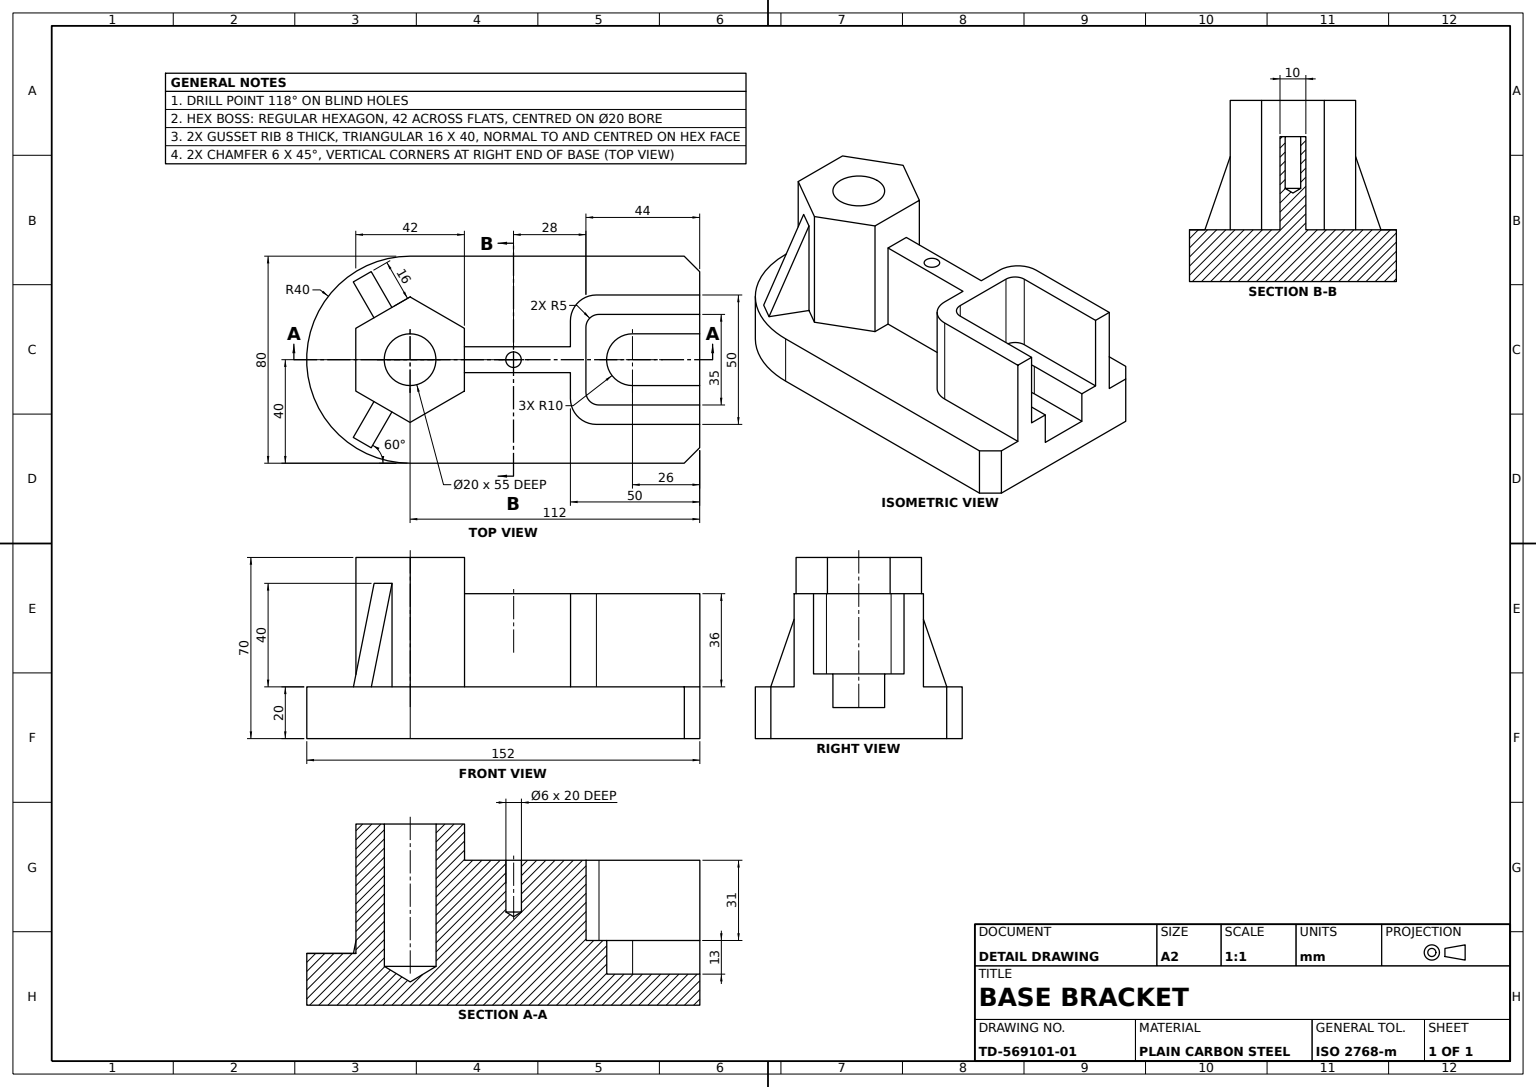
ISO-10303-21;
HEADER;
FILE_DESCRIPTION((''),'2;1');
FILE_NAME('','',(''),(''),'','','');
FILE_SCHEMA(('AUTOMOTIVE_DESIGN'));
ENDSEC;
DATA;
#1=APPLICATION_CONTEXT('');
#2=PRODUCT_CONTEXT('',#1,'mechanical');
#3=PRODUCT('','','',(#2));
#4=PRODUCT_DEFINITION_FORMATION('','',#3);
#5=PRODUCT_DEFINITION_CONTEXT('',#1,'design');
#6=PRODUCT_DEFINITION('','',#4,#5);
#7=PRODUCT_DEFINITION_SHAPE('','',#6);
#8=(LENGTH_UNIT()NAMED_UNIT(*)SI_UNIT(.MILLI.,.METRE.));
#9=(NAMED_UNIT(*)PLANE_ANGLE_UNIT()SI_UNIT($,.RADIAN.));
#10=(NAMED_UNIT(*)SI_UNIT($,.STERADIAN.)SOLID_ANGLE_UNIT());
#11=UNCERTAINTY_MEASURE_WITH_UNIT(LENGTH_MEASURE(1.E-05),#8,'distance_accuracy_value','');
#12=(GEOMETRIC_REPRESENTATION_CONTEXT(3)GLOBAL_UNCERTAINTY_ASSIGNED_CONTEXT((#11))GLOBAL_UNIT_ASSIGNED_CONTEXT((#8,#9,#10))REPRESENTATION_CONTEXT('',''));
#13=CARTESIAN_POINT('',(112.,12.,10.));
#14=VERTEX_POINT('',#13);
#15=CARTESIAN_POINT('',(112.,12.,-10.));
#16=VERTEX_POINT('',#15);
#17=DIRECTION('',(0.,0.,-1.));
#18=VECTOR('',#17,1000.);
#19=LINE('',#15,#18);
#20=EDGE_CURVE('',#14,#16,#19,.T.);
#21=ORIENTED_EDGE('',*,*,#20,.T.);
#22=CARTESIAN_POINT('',(86.,12.,-10.));
#23=VERTEX_POINT('',#22);
#24=DIRECTION('',(-1.,0.,0.));
#25=VECTOR('',#24,1000.);
#26=LINE('',#22,#25);
#27=EDGE_CURVE('',#16,#23,#26,.T.);
#28=ORIENTED_EDGE('',*,*,#27,.T.);
#29=CARTESIAN_POINT('',(86.,12.,10.));
#30=VERTEX_POINT('',#29);
#31=CARTESIAN_POINT('',(86.,12.,0.));
#32=DIRECTION('',(0.,1.,0.));
#33=DIRECTION('',(0.,0.,1.));
#34=AXIS2_PLACEMENT_3D('',#31,#32,#33);
#35=CIRCLE('',#34,10.);
#36=EDGE_CURVE('',#23,#30,#35,.T.);
#37=ORIENTED_EDGE('',*,*,#36,.T.);
#38=DIRECTION('',(1.,0.,0.));
#39=VECTOR('',#38,1000.);
#40=LINE('',#13,#39);
#41=EDGE_CURVE('',#30,#14,#40,.T.);
#42=ORIENTED_EDGE('',*,*,#41,.T.);
#43=EDGE_LOOP('',(#21,#28,#37,#42));
#44=FACE_OUTER_BOUND('',#43,.T.);
#45=PLANE('',#34);
#46=ADVANCED_FACE('',(#44),#45,.T.);
#47=CARTESIAN_POINT('',(62.,56.,5.));
#48=VERTEX_POINT('',#47);
#49=CARTESIAN_POINT('',(62.,20.,5.));
#50=VERTEX_POINT('',#49);
#51=DIRECTION('',(0.,-1.,0.));
#52=VECTOR('',#51,1000.);
#53=LINE('',#47,#52);
#54=EDGE_CURVE('',#48,#50,#53,.T.);
#55=ORIENTED_EDGE('',*,*,#54,.T.);
#56=CARTESIAN_POINT('',(62.,20.,15.));
#57=VERTEX_POINT('',#56);
#58=VECTOR('',#33,1000.);
#59=LINE('',#49,#58);
#60=EDGE_CURVE('',#50,#57,#59,.T.);
#61=ORIENTED_EDGE('',*,*,#60,.T.);
#62=CARTESIAN_POINT('',(62.,56.,15.));
#63=VERTEX_POINT('',#62);
#64=VECTOR('',#32,1000.);
#65=LINE('',#62,#64);
#66=EDGE_CURVE('',#57,#63,#65,.T.);
#67=ORIENTED_EDGE('',*,*,#66,.T.);
#68=LINE('',#47,#58);
#69=EDGE_CURVE('',#48,#63,#68,.T.);
#70=ORIENTED_EDGE('',*,*,#69,.F.);
#71=EDGE_LOOP('',(#55,#61,#67,#70));
#72=FACE_OUTER_BOUND('',#71,.T.);
#73=AXIS2_PLACEMENT_3D('',#47,#38,#17);
#74=PLANE('',#73);
#75=ADVANCED_FACE('',(#72),#74,.F.);
#76=CARTESIAN_POINT('',(106.,0.,40.));
#77=VERTEX_POINT('',#76);
#78=CARTESIAN_POINT('',(112.,0.,34.));
#79=VERTEX_POINT('',#78);
#80=DIRECTION('',(0.707106781,0.,-0.707106781));
#81=VECTOR('',#80,1000.);
#82=LINE('',#78,#81);
#83=EDGE_CURVE('',#77,#79,#82,.T.);
#84=ORIENTED_EDGE('',*,*,#83,.T.);
#85=CARTESIAN_POINT('',(112.,20.,34.));
#86=VERTEX_POINT('',#85);
#87=LINE('',#85,#52);
#88=EDGE_CURVE('',#86,#79,#87,.T.);
#89=ORIENTED_EDGE('',*,*,#88,.F.);
#90=CARTESIAN_POINT('',(106.,20.,40.));
#91=VERTEX_POINT('',#90);
#92=LINE('',#85,#81);
#93=EDGE_CURVE('',#91,#86,#92,.T.);
#94=ORIENTED_EDGE('',*,*,#93,.F.);
#95=LINE('',#90,#52);
#96=EDGE_CURVE('',#91,#77,#95,.T.);
#97=ORIENTED_EDGE('',*,*,#96,.T.);
#98=EDGE_LOOP('',(#84,#89,#94,#97));
#99=FACE_OUTER_BOUND('',#98,.T.);
#100=DIRECTION('',(-0.707106781,0.,-0.707106781));
#101=DIRECTION('',(-0.707106781,0.,0.707106781));
#102=AXIS2_PLACEMENT_3D('',#85,#100,#101);
#103=PLANE('',#102);
#104=ADVANCED_FACE('',(#99),#103,.F.);
#105=CARTESIAN_POINT('',(73.,25.,-17.5));
#106=VERTEX_POINT('',#105);
#107=CARTESIAN_POINT('',(73.,56.,-17.5));
#108=VERTEX_POINT('',#107);
#109=LINE('',#105,#64);
#110=EDGE_CURVE('',#106,#108,#109,.T.);
#111=ORIENTED_EDGE('',*,*,#110,.F.);
#112=CARTESIAN_POINT('',(112.,25.,-17.5));
#113=VERTEX_POINT('',#112);
#114=LINE('',#112,#25);
#115=EDGE_CURVE('',#113,#106,#114,.T.);
#116=ORIENTED_EDGE('',*,*,#115,.F.);
#117=CARTESIAN_POINT('',(112.,56.,-17.5));
#118=VERTEX_POINT('',#117);
#119=LINE('',#112,#64);
#120=EDGE_CURVE('',#113,#118,#119,.T.);
#121=ORIENTED_EDGE('',*,*,#120,.T.);
#122=LINE('',#117,#25);
#123=EDGE_CURVE('',#118,#108,#122,.T.);
#124=ORIENTED_EDGE('',*,*,#123,.T.);
#125=EDGE_LOOP('',(#111,#116,#121,#124));
#126=FACE_OUTER_BOUND('',#125,.T.);
#127=AXIS2_PLACEMENT_3D('',#112,#17,#24);
#128=PLANE('',#127);
#129=ADVANCED_FACE('',(#126),#128,.F.);
#130=CARTESIAN_POINT('',(21.,56.,-5.));
#131=VERTEX_POINT('',#130);
#132=CARTESIAN_POINT('',(21.,20.,-5.));
#133=VERTEX_POINT('',#132);
#134=LINE('',#130,#52);
#135=EDGE_CURVE('',#131,#133,#134,.T.);
#136=ORIENTED_EDGE('',*,*,#135,.F.);
#137=CARTESIAN_POINT('',(62.,56.,-5.));
#138=VERTEX_POINT('',#137);
#139=LINE('',#130,#25);
#140=EDGE_CURVE('',#138,#131,#139,.T.);
#141=ORIENTED_EDGE('',*,*,#140,.F.);
#142=CARTESIAN_POINT('',(62.,20.,-5.));
#143=VERTEX_POINT('',#142);
#144=LINE('',#137,#52);
#145=EDGE_CURVE('',#138,#143,#144,.T.);
#146=ORIENTED_EDGE('',*,*,#145,.T.);
#147=LINE('',#132,#25);
#148=EDGE_CURVE('',#143,#133,#147,.T.);
#149=ORIENTED_EDGE('',*,*,#148,.T.);
#150=EDGE_LOOP('',(#136,#141,#146,#149));
#151=FACE_OUTER_BOUND('',#150,.T.);
#152=AXIS2_PLACEMENT_3D('',#130,#33,#38);
#153=PLANE('',#152);
#154=ADVANCED_FACE('',(#151),#153,.F.);
#155=CARTESIAN_POINT('',(-21.964102,20.,-30.04294));
#156=VERTEX_POINT('',#155);
#157=CARTESIAN_POINT('',(-13.964102,60.,-16.186533));
#158=VERTEX_POINT('',#157);
#159=DIRECTION('',(0.185695338,0.928476691,0.32163376));
#160=VECTOR('',#159,1000.);
#161=LINE('',#157,#160);
#162=EDGE_CURVE('',#156,#158,#161,.T.);
#163=ORIENTED_EDGE('',*,*,#162,.T.);
#164=CARTESIAN_POINT('',(-7.035898,60.,-20.186533));
#165=VERTEX_POINT('',#164);
#166=DIRECTION('',(0.866025404,0.,-0.5));
#167=VECTOR('',#166,1000.);
#168=LINE('',#164,#167);
#169=EDGE_CURVE('',#158,#165,#168,.T.);
#170=ORIENTED_EDGE('',*,*,#169,.T.);
#171=CARTESIAN_POINT('',(-15.035898,20.,-34.04294));
#172=VERTEX_POINT('',#171);
#173=CARTESIAN_POINT('',(-8.139347,54.482759,-22.097762));
#174=LINE('',#173,#160);
#175=EDGE_CURVE('',#172,#165,#174,.T.);
#176=ORIENTED_EDGE('',*,*,#175,.F.);
#177=DIRECTION('',(-0.866025404,0.,0.5));
#178=VECTOR('',#177,1000.);
#179=LINE('',#171,#178);
#180=EDGE_CURVE('',#172,#156,#179,.T.);
#181=ORIENTED_EDGE('',*,*,#180,.T.);
#182=EDGE_LOOP('',(#163,#170,#176,#181));
#183=FACE_OUTER_BOUND('',#182,.T.);
#184=CARTESIAN_POINT('',(-0.107695,60.,-24.186533));
#185=DIRECTION('',(0.464238345,-0.371390676,0.804084401));
#186=AXIS2_PLACEMENT_3D('',#184,#185,#166);
#187=PLANE('',#186);
#188=ADVANCED_FACE('',(#183),#187,.F.);
#189=CARTESIAN_POINT('',(0.,15.,10.));
#190=VERTEX_POINT('',#189);
#191=CARTESIAN_POINT('',(0.,70.,10.));
#192=VERTEX_POINT('',#191);
#193=LINE('',#191,#64);
#194=EDGE_CURVE('',#190,#192,#193,.T.);
#195=ORIENTED_EDGE('',*,*,#194,.F.);
#196=CARTESIAN_POINT('',(0.,15.,-10.));
#197=VERTEX_POINT('',#196);
#198=CARTESIAN_POINT('',(0.,15.,0.));
#199=AXIS2_PLACEMENT_3D('',#198,#32,#33);
#200=CIRCLE('',#199,10.);
#201=EDGE_CURVE('',#197,#190,#200,.T.);
#202=ORIENTED_EDGE('',*,*,#201,.F.);
#203=CARTESIAN_POINT('',(0.,70.,-10.));
#204=VERTEX_POINT('',#203);
#205=LINE('',#203,#64);
#206=EDGE_CURVE('',#197,#204,#205,.T.);
#207=ORIENTED_EDGE('',*,*,#206,.T.);
#208=CARTESIAN_POINT('',(0.,70.,0.));
#209=AXIS2_PLACEMENT_3D('',#208,#32,#33);
#210=CIRCLE('',#209,10.);
#211=EDGE_CURVE('',#204,#192,#210,.T.);
#212=ORIENTED_EDGE('',*,*,#211,.T.);
#213=EDGE_LOOP('',(#195,#202,#207,#212));
#214=FACE_OUTER_BOUND('',#213,.T.);
#215=CYLINDRICAL_SURFACE('',#209,10.);
#216=ADVANCED_FACE('',(#214),#215,.F.);
#217=CARTESIAN_POINT('',(0.,8.991394,0.));
#218=VERTEX_POINT('',#217);
#219=DIRECTION('',(0.,0.515038075,-0.857167301));
#220=VECTOR('',#219,1000.);
#221=LINE('',#196,#220);
#222=EDGE_CURVE('',#218,#197,#221,.T.);
#223=ORIENTED_EDGE('',*,*,#222,.T.);
#224=ORIENTED_EDGE('',*,*,#201,.T.);
#225=DIRECTION('',(0.,0.515038075,0.857167301));
#226=VECTOR('',#225,1000.);
#227=LINE('',#189,#226);
#228=EDGE_CURVE('',#218,#190,#227,.T.);
#229=ORIENTED_EDGE('',*,*,#228,.F.);
#230=EDGE_LOOP('',(#223,#224,#229));
#231=FACE_OUTER_BOUND('',#230,.T.);
#232=CONICAL_SURFACE('',#199,10.,1.029744259);
#233=ADVANCED_FACE('',(#231),#232,.F.);
#234=CARTESIAN_POINT('',(0.,70.,24.248711));
#235=VERTEX_POINT('',#234);
#236=CARTESIAN_POINT('',(0.,20.,24.248711));
#237=VERTEX_POINT('',#236);
#238=LINE('',#234,#52);
#239=EDGE_CURVE('',#235,#237,#238,.T.);
#240=ORIENTED_EDGE('',*,*,#239,.T.);
#241=CARTESIAN_POINT('',(21.,20.,12.124356));
#242=VERTEX_POINT('',#241);
#243=LINE('',#236,#167);
#244=EDGE_CURVE('',#237,#242,#243,.T.);
#245=ORIENTED_EDGE('',*,*,#244,.T.);
#246=CARTESIAN_POINT('',(21.,70.,12.124356));
#247=VERTEX_POINT('',#246);
#248=LINE('',#246,#52);
#249=EDGE_CURVE('',#247,#242,#248,.T.);
#250=ORIENTED_EDGE('',*,*,#249,.F.);
#251=LINE('',#234,#167);
#252=EDGE_CURVE('',#235,#247,#251,.T.);
#253=ORIENTED_EDGE('',*,*,#252,.F.);
#254=EDGE_LOOP('',(#240,#245,#250,#253));
#255=FACE_OUTER_BOUND('',#254,.T.);
#256=DIRECTION('',(-0.5,0.,-0.866025404));
#257=AXIS2_PLACEMENT_3D('',#234,#256,#177);
#258=PLANE('',#257);
#259=ADVANCED_FACE('',(#255),#258,.F.);
#260=CARTESIAN_POINT('',(0.,20.,-40.));
#261=VERTEX_POINT('',#260);
#262=CARTESIAN_POINT('',(0.,0.,-40.));
#263=VERTEX_POINT('',#262);
#264=LINE('',#260,#52);
#265=EDGE_CURVE('',#261,#263,#264,.T.);
#266=ORIENTED_EDGE('',*,*,#265,.T.);
#267=CARTESIAN_POINT('',(0.,0.,40.));
#268=VERTEX_POINT('',#267);
#269=CARTESIAN_POINT('',(0.,0.,0.));
#270=AXIS2_PLACEMENT_3D('',#269,#32,#33);
#271=CIRCLE('',#270,40.);
#272=EDGE_CURVE('',#263,#268,#271,.T.);
#273=ORIENTED_EDGE('',*,*,#272,.T.);
#274=CARTESIAN_POINT('',(0.,20.,40.));
#275=VERTEX_POINT('',#274);
#276=LINE('',#274,#52);
#277=EDGE_CURVE('',#275,#268,#276,.T.);
#278=ORIENTED_EDGE('',*,*,#277,.F.);
#279=CARTESIAN_POINT('',(0.,20.,0.));
#280=AXIS2_PLACEMENT_3D('',#279,#32,#33);
#281=CIRCLE('',#280,40.);
#282=EDGE_CURVE('',#261,#275,#281,.T.);
#283=ORIENTED_EDGE('',*,*,#282,.F.);
#284=EDGE_LOOP('',(#266,#273,#278,#283));
#285=FACE_OUTER_BOUND('',#284,.T.);
#286=AXIS2_PLACEMENT_3D('',#279,#51,#17);
#287=CYLINDRICAL_SURFACE('',#286,40.);
#288=ADVANCED_FACE('',(#285),#287,.T.);
#289=CARTESIAN_POINT('',(21.,20.,5.));
#290=VERTEX_POINT('',#289);
#291=LINE('',#289,#39);
#292=EDGE_CURVE('',#290,#50,#291,.T.);
#293=ORIENTED_EDGE('',*,*,#292,.T.);
#294=ORIENTED_EDGE('',*,*,#54,.F.);
#295=CARTESIAN_POINT('',(21.,56.,5.));
#296=VERTEX_POINT('',#295);
#297=LINE('',#295,#39);
#298=EDGE_CURVE('',#296,#48,#297,.T.);
#299=ORIENTED_EDGE('',*,*,#298,.F.);
#300=LINE('',#295,#52);
#301=EDGE_CURVE('',#296,#290,#300,.T.);
#302=ORIENTED_EDGE('',*,*,#301,.T.);
#303=EDGE_LOOP('',(#293,#294,#299,#302));
#304=FACE_OUTER_BOUND('',#303,.T.);
#305=AXIS2_PLACEMENT_3D('',#295,#17,#24);
#306=PLANE('',#305);
#307=ADVANCED_FACE('',(#304),#306,.F.);
#308=EDGE_CURVE('',#192,#204,#210,.T.);
#309=ORIENTED_EDGE('',*,*,#308,.T.);
#310=ORIENTED_EDGE('',*,*,#206,.F.);
#311=EDGE_CURVE('',#190,#197,#200,.T.);
#312=ORIENTED_EDGE('',*,*,#311,.F.);
#313=ORIENTED_EDGE('',*,*,#194,.T.);
#314=EDGE_LOOP('',(#309,#310,#312,#313));
#315=FACE_OUTER_BOUND('',#314,.T.);
#316=ADVANCED_FACE('',(#315),#215,.F.);
#317=CARTESIAN_POINT('',(68.,25.,12.5));
#318=VERTEX_POINT('',#317);
#319=CARTESIAN_POINT('',(73.,25.,17.5));
#320=VERTEX_POINT('',#319);
#321=CARTESIAN_POINT('',(73.,25.,12.5));
#322=AXIS2_PLACEMENT_3D('',#321,#32,#33);
#323=CIRCLE('',#322,5.);
#324=EDGE_CURVE('',#318,#320,#323,.T.);
#325=ORIENTED_EDGE('',*,*,#324,.F.);
#326=CARTESIAN_POINT('',(68.,56.,12.5));
#327=VERTEX_POINT('',#326);
#328=LINE('',#317,#64);
#329=EDGE_CURVE('',#318,#327,#328,.T.);
#330=ORIENTED_EDGE('',*,*,#329,.T.);
#331=CARTESIAN_POINT('',(73.,56.,17.5));
#332=VERTEX_POINT('',#331);
#333=CARTESIAN_POINT('',(73.,56.,12.5));
#334=AXIS2_PLACEMENT_3D('',#333,#32,#33);
#335=CIRCLE('',#334,5.);
#336=EDGE_CURVE('',#327,#332,#335,.T.);
#337=ORIENTED_EDGE('',*,*,#336,.T.);
#338=LINE('',#319,#64);
#339=EDGE_CURVE('',#320,#332,#338,.T.);
#340=ORIENTED_EDGE('',*,*,#339,.F.);
#341=EDGE_LOOP('',(#325,#330,#337,#340));
#342=FACE_OUTER_BOUND('',#341,.T.);
#343=CYLINDRICAL_SURFACE('',#322,5.);
#344=ADVANCED_FACE('',(#342),#343,.F.);
#345=CARTESIAN_POINT('',(112.,0.,-34.));
#346=VERTEX_POINT('',#345);
#347=CARTESIAN_POINT('',(106.,0.,-40.));
#348=VERTEX_POINT('',#347);
#349=VECTOR('',#100,1000.);
#350=LINE('',#347,#349);
#351=EDGE_CURVE('',#346,#348,#350,.T.);
#352=ORIENTED_EDGE('',*,*,#351,.T.);
#353=CARTESIAN_POINT('',(106.,20.,-40.));
#354=VERTEX_POINT('',#353);
#355=LINE('',#353,#52);
#356=EDGE_CURVE('',#354,#348,#355,.T.);
#357=ORIENTED_EDGE('',*,*,#356,.F.);
#358=CARTESIAN_POINT('',(112.,20.,-34.));
#359=VERTEX_POINT('',#358);
#360=LINE('',#353,#349);
#361=EDGE_CURVE('',#359,#354,#360,.T.);
#362=ORIENTED_EDGE('',*,*,#361,.F.);
#363=LINE('',#358,#52);
#364=EDGE_CURVE('',#359,#346,#363,.T.);
#365=ORIENTED_EDGE('',*,*,#364,.T.);
#366=EDGE_LOOP('',(#352,#357,#362,#365));
#367=FACE_OUTER_BOUND('',#366,.T.);
#368=DIRECTION('',(0.707106781,0.,0.707106781));
#369=AXIS2_PLACEMENT_3D('',#353,#101,#368);
#370=PLANE('',#369);
#371=ADVANCED_FACE('',(#367),#370,.F.);
#372=ORIENTED_EDGE('',*,*,#311,.T.);
#373=ORIENTED_EDGE('',*,*,#222,.F.);
#374=ORIENTED_EDGE('',*,*,#228,.T.);
#375=EDGE_LOOP('',(#372,#373,#374));
#376=FACE_OUTER_BOUND('',#375,.T.);
#377=ADVANCED_FACE('',(#376),#232,.F.);
#378=CARTESIAN_POINT('',(40.,34.197418,0.));
#379=VERTEX_POINT('',#378);
#380=CARTESIAN_POINT('',(40.,36.,-3.));
#381=VERTEX_POINT('',#380);
#382=LINE('',#380,#220);
#383=EDGE_CURVE('',#379,#381,#382,.T.);
#384=ORIENTED_EDGE('',*,*,#383,.F.);
#385=CARTESIAN_POINT('',(40.,36.,3.));
#386=VERTEX_POINT('',#385);
#387=LINE('',#385,#226);
#388=EDGE_CURVE('',#379,#386,#387,.T.);
#389=ORIENTED_EDGE('',*,*,#388,.T.);
#390=CARTESIAN_POINT('',(40.,36.,0.));
#391=AXIS2_PLACEMENT_3D('',#390,#32,#33);
#392=CIRCLE('',#391,3.);
#393=EDGE_CURVE('',#386,#381,#392,.T.);
#394=ORIENTED_EDGE('',*,*,#393,.T.);
#395=EDGE_LOOP('',(#384,#389,#394));
#396=FACE_OUTER_BOUND('',#395,.T.);
#397=CONICAL_SURFACE('',#391,3.,1.029744259);
#398=ADVANCED_FACE('',(#396),#397,.F.);
#399=CARTESIAN_POINT('',(-21.,70.,12.124356));
#400=VERTEX_POINT('',#399);
#401=DIRECTION('',(0.866025404,0.,0.5));
#402=VECTOR('',#401,1000.);
#403=LINE('',#399,#402);
#404=EDGE_CURVE('',#400,#235,#403,.T.);
#405=ORIENTED_EDGE('',*,*,#404,.T.);
#406=ORIENTED_EDGE('',*,*,#252,.T.);
#407=CARTESIAN_POINT('',(21.,70.,-12.124356));
#408=VERTEX_POINT('',#407);
#409=LINE('',#246,#18);
#410=EDGE_CURVE('',#247,#408,#409,.T.);
#411=ORIENTED_EDGE('',*,*,#410,.T.);
#412=CARTESIAN_POINT('',(0.,70.,-24.248711));
#413=VERTEX_POINT('',#412);
#414=DIRECTION('',(-0.866025404,0.,-0.5));
#415=VECTOR('',#414,1000.);
#416=LINE('',#407,#415);
#417=EDGE_CURVE('',#408,#413,#416,.T.);
#418=ORIENTED_EDGE('',*,*,#417,.T.);
#419=CARTESIAN_POINT('',(-21.,70.,-12.124356));
#420=VERTEX_POINT('',#419);
#421=LINE('',#412,#178);
#422=EDGE_CURVE('',#413,#420,#421,.T.);
#423=ORIENTED_EDGE('',*,*,#422,.T.);
#424=LINE('',#419,#58);
#425=EDGE_CURVE('',#420,#400,#424,.T.);
#426=ORIENTED_EDGE('',*,*,#425,.T.);
#427=EDGE_LOOP('',(#405,#406,#411,#418,#423,#426));
#428=FACE_OUTER_BOUND('',#427,.T.);
#429=ORIENTED_EDGE('',*,*,#211,.F.);
#430=ORIENTED_EDGE('',*,*,#308,.F.);
#431=EDGE_LOOP('',(#429,#430));
#432=FACE_BOUND('',#431,.T.);
#433=PLANE('',#209);
#434=ADVANCED_FACE('',(#428,#432),#433,.T.);
#435=ORIENTED_EDGE('',*,*,#272,.F.);
#436=LINE('',#262,#25);
#437=EDGE_CURVE('',#348,#263,#436,.T.);
#438=ORIENTED_EDGE('',*,*,#437,.F.);
#439=ORIENTED_EDGE('',*,*,#351,.F.);
#440=LINE('',#345,#18);
#441=EDGE_CURVE('',#79,#346,#440,.T.);
#442=ORIENTED_EDGE('',*,*,#441,.F.);
#443=ORIENTED_EDGE('',*,*,#83,.F.);
#444=LINE('',#76,#39);
#445=EDGE_CURVE('',#268,#77,#444,.T.);
#446=ORIENTED_EDGE('',*,*,#445,.F.);
#447=EDGE_LOOP('',(#435,#438,#439,#442,#443,#446));
#448=FACE_OUTER_BOUND('',#447,.T.);
#449=PLANE('',#270);
#450=ADVANCED_FACE('',(#448),#449,.F.);
#451=CARTESIAN_POINT('',(-21.964102,20.,30.04294));
#452=VERTEX_POINT('',#451);
#453=CARTESIAN_POINT('',(-15.035898,20.,34.04294));
#454=VERTEX_POINT('',#453);
#455=LINE('',#451,#402);
#456=EDGE_CURVE('',#452,#454,#455,.T.);
#457=ORIENTED_EDGE('',*,*,#456,.T.);
#458=CARTESIAN_POINT('',(-7.035898,60.,20.186533));
#459=VERTEX_POINT('',#458);
#460=DIRECTION('',(0.185695338,0.928476691,-0.32163376));
#461=VECTOR('',#460,1000.);
#462=LINE('',#458,#461);
#463=EDGE_CURVE('',#454,#459,#462,.T.);
#464=ORIENTED_EDGE('',*,*,#463,.T.);
#465=CARTESIAN_POINT('',(-13.964102,60.,16.186533));
#466=VERTEX_POINT('',#465);
#467=LINE('',#465,#415);
#468=EDGE_CURVE('',#459,#466,#467,.T.);
#469=ORIENTED_EDGE('',*,*,#468,.T.);
#470=CARTESIAN_POINT('',(-15.06755,54.482759,18.097762));
#471=LINE('',#470,#461);
#472=EDGE_CURVE('',#452,#466,#471,.T.);
#473=ORIENTED_EDGE('',*,*,#472,.F.);
#474=EDGE_LOOP('',(#457,#464,#469,#473));
#475=FACE_OUTER_BOUND('',#474,.T.);
#476=CARTESIAN_POINT('',(-20.892305,60.,12.186533));
#477=DIRECTION('',(0.464238345,-0.371390676,-0.804084401));
#478=AXIS2_PLACEMENT_3D('',#476,#477,#414);
#479=PLANE('',#478);
#480=ADVANCED_FACE('',(#475),#479,.F.);
#481=CARTESIAN_POINT('',(40.,56.,-3.));
#482=VERTEX_POINT('',#481);
#483=CARTESIAN_POINT('',(40.,56.,3.));
#484=VERTEX_POINT('',#483);
#485=CARTESIAN_POINT('',(40.,56.,0.));
#486=AXIS2_PLACEMENT_3D('',#485,#32,#33);
#487=CIRCLE('',#486,3.);
#488=EDGE_CURVE('',#482,#484,#487,.T.);
#489=ORIENTED_EDGE('',*,*,#488,.T.);
#490=LINE('',#483,#64);
#491=EDGE_CURVE('',#386,#484,#490,.T.);
#492=ORIENTED_EDGE('',*,*,#491,.F.);
#493=EDGE_CURVE('',#381,#386,#392,.T.);
#494=ORIENTED_EDGE('',*,*,#493,.F.);
#495=LINE('',#481,#64);
#496=EDGE_CURVE('',#381,#482,#495,.T.);
#497=ORIENTED_EDGE('',*,*,#496,.T.);
#498=EDGE_LOOP('',(#489,#492,#494,#497));
#499=FACE_OUTER_BOUND('',#498,.T.);
#500=CYLINDRICAL_SURFACE('',#486,3.);
#501=ADVANCED_FACE('',(#499),#500,.F.);
#502=ORIENTED_EDGE('',*,*,#463,.F.);
#503=CARTESIAN_POINT('',(-7.035898,20.,20.186533));
#504=VERTEX_POINT('',#503);
#505=DIRECTION('',(0.5,0.,-0.866025404));
#506=VECTOR('',#505,1000.);
#507=LINE('',#453,#506);
#508=EDGE_CURVE('',#454,#504,#507,.T.);
#509=ORIENTED_EDGE('',*,*,#508,.T.);
#510=LINE('',#458,#64);
#511=EDGE_CURVE('',#504,#459,#510,.T.);
#512=ORIENTED_EDGE('',*,*,#511,.T.);
#513=EDGE_LOOP('',(#502,#509,#512));
#514=FACE_OUTER_BOUND('',#513,.T.);
#515=CARTESIAN_POINT('',(-15.035898,60.,34.04294));
#516=DIRECTION('',(-0.5,0.,0.866025404));
#517=AXIS2_PLACEMENT_3D('',#515,#414,#516);
#518=PLANE('',#517);
#519=ADVANCED_FACE('',(#514),#518,.F.);
#520=ORIENTED_EDGE('',*,*,#239,.F.);
#521=ORIENTED_EDGE('',*,*,#404,.F.);
#522=CARTESIAN_POINT('',(-21.,20.,12.124356));
#523=VERTEX_POINT('',#522);
#524=LINE('',#399,#52);
#525=EDGE_CURVE('',#400,#523,#524,.T.);
#526=ORIENTED_EDGE('',*,*,#525,.T.);
#527=CARTESIAN_POINT('',(-13.964102,20.,16.186533));
#528=VERTEX_POINT('',#527);
#529=LINE('',#522,#402);
#530=EDGE_CURVE('',#523,#528,#529,.T.);
#531=ORIENTED_EDGE('',*,*,#530,.T.);
#532=LINE('',#465,#52);
#533=EDGE_CURVE('',#466,#528,#532,.T.);
#534=ORIENTED_EDGE('',*,*,#533,.F.);
#535=ORIENTED_EDGE('',*,*,#468,.F.);
#536=ORIENTED_EDGE('',*,*,#511,.F.);
#537=EDGE_CURVE('',#504,#237,#529,.T.);
#538=ORIENTED_EDGE('',*,*,#537,.T.);
#539=EDGE_LOOP('',(#520,#521,#526,#531,#534,#535,#536,#538));
#540=FACE_OUTER_BOUND('',#539,.T.);
#541=AXIS2_PLACEMENT_3D('',#399,#505,#414);
#542=PLANE('',#541);
#543=ADVANCED_FACE('',(#540),#542,.F.);
#544=ORIENTED_EDGE('',*,*,#437,.T.);
#545=ORIENTED_EDGE('',*,*,#265,.F.);
#546=LINE('',#260,#25);
#547=EDGE_CURVE('',#354,#261,#546,.T.);
#548=ORIENTED_EDGE('',*,*,#547,.F.);
#549=ORIENTED_EDGE('',*,*,#356,.T.);
#550=EDGE_LOOP('',(#544,#545,#548,#549));
#551=FACE_OUTER_BOUND('',#550,.T.);
#552=AXIS2_PLACEMENT_3D('',#260,#33,#38);
#553=PLANE('',#552);
#554=ADVANCED_FACE('',(#551),#553,.F.);
#555=LINE('',#90,#39);
#556=EDGE_CURVE('',#275,#91,#555,.T.);
#557=ORIENTED_EDGE('',*,*,#556,.F.);
#558=ORIENTED_EDGE('',*,*,#277,.T.);
#559=ORIENTED_EDGE('',*,*,#445,.T.);
#560=ORIENTED_EDGE('',*,*,#96,.F.);
#561=EDGE_LOOP('',(#557,#558,#559,#560));
#562=FACE_OUTER_BOUND('',#561,.T.);
#563=AXIS2_PLACEMENT_3D('',#90,#17,#24);
#564=PLANE('',#563);
#565=ADVANCED_FACE('',(#562),#564,.F.);
#566=LINE('',#451,#506);
#567=EDGE_CURVE('',#452,#528,#566,.T.);
#568=ORIENTED_EDGE('',*,*,#567,.F.);
#569=ORIENTED_EDGE('',*,*,#472,.T.);
#570=ORIENTED_EDGE('',*,*,#533,.T.);
#571=EDGE_LOOP('',(#568,#569,#570));
#572=FACE_OUTER_BOUND('',#571,.T.);
#573=CARTESIAN_POINT('',(-21.964102,60.,30.04294));
#574=AXIS2_PLACEMENT_3D('',#573,#401,#505);
#575=PLANE('',#574);
#576=ADVANCED_FACE('',(#572),#575,.F.);
#577=CARTESIAN_POINT('',(86.,25.,10.));
#578=VERTEX_POINT('',#577);
#579=CARTESIAN_POINT('',(112.,25.,10.));
#580=VERTEX_POINT('',#579);
#581=LINE('',#579,#39);
#582=EDGE_CURVE('',#578,#580,#581,.T.);
#583=ORIENTED_EDGE('',*,*,#582,.T.);
#584=LINE('',#13,#64);
#585=EDGE_CURVE('',#14,#580,#584,.T.);
#586=ORIENTED_EDGE('',*,*,#585,.F.);
#587=ORIENTED_EDGE('',*,*,#41,.F.);
#588=LINE('',#29,#64);
#589=EDGE_CURVE('',#30,#578,#588,.T.);
#590=ORIENTED_EDGE('',*,*,#589,.T.);
#591=EDGE_LOOP('',(#583,#586,#587,#590));
#592=FACE_OUTER_BOUND('',#591,.T.);
#593=AXIS2_PLACEMENT_3D('',#13,#33,#38);
#594=PLANE('',#593);
#595=ADVANCED_FACE('',(#592),#594,.F.);
#596=ORIENTED_EDGE('',*,*,#88,.T.);
#597=ORIENTED_EDGE('',*,*,#441,.T.);
#598=ORIENTED_EDGE('',*,*,#364,.F.);
#599=CARTESIAN_POINT('',(112.,20.,-25.));
#600=VERTEX_POINT('',#599);
#601=LINE('',#358,#18);
#602=EDGE_CURVE('',#600,#359,#601,.T.);
#603=ORIENTED_EDGE('',*,*,#602,.F.);
#604=CARTESIAN_POINT('',(112.,56.,-25.));
#605=VERTEX_POINT('',#604);
#606=LINE('',#604,#52);
#607=EDGE_CURVE('',#605,#600,#606,.T.);
#608=ORIENTED_EDGE('',*,*,#607,.F.);
#609=LINE('',#604,#18);
#610=EDGE_CURVE('',#118,#605,#609,.T.);
#611=ORIENTED_EDGE('',*,*,#610,.F.);
#612=ORIENTED_EDGE('',*,*,#120,.F.);
#613=CARTESIAN_POINT('',(112.,25.,-10.));
#614=VERTEX_POINT('',#613);
#615=LINE('',#112,#18);
#616=EDGE_CURVE('',#614,#113,#615,.T.);
#617=ORIENTED_EDGE('',*,*,#616,.F.);
#618=LINE('',#15,#64);
#619=EDGE_CURVE('',#16,#614,#618,.T.);
#620=ORIENTED_EDGE('',*,*,#619,.F.);
#621=ORIENTED_EDGE('',*,*,#20,.F.);
#622=ORIENTED_EDGE('',*,*,#585,.T.);
#623=CARTESIAN_POINT('',(112.,25.,17.5));
#624=VERTEX_POINT('',#623);
#625=EDGE_CURVE('',#624,#580,#615,.T.);
#626=ORIENTED_EDGE('',*,*,#625,.F.);
#627=CARTESIAN_POINT('',(112.,56.,17.5));
#628=VERTEX_POINT('',#627);
#629=LINE('',#623,#64);
#630=EDGE_CURVE('',#624,#628,#629,.T.);
#631=ORIENTED_EDGE('',*,*,#630,.T.);
#632=CARTESIAN_POINT('',(112.,56.,25.));
#633=VERTEX_POINT('',#632);
#634=EDGE_CURVE('',#633,#628,#609,.T.);
#635=ORIENTED_EDGE('',*,*,#634,.F.);
#636=CARTESIAN_POINT('',(112.,20.,25.));
#637=VERTEX_POINT('',#636);
#638=LINE('',#632,#52);
#639=EDGE_CURVE('',#633,#637,#638,.T.);
#640=ORIENTED_EDGE('',*,*,#639,.T.);
#641=EDGE_CURVE('',#86,#637,#601,.T.);
#642=ORIENTED_EDGE('',*,*,#641,.F.);
#643=EDGE_LOOP('',(#596,#597,#598,#603,#608,#611,#612,#617,#620,#621,#622,#626,#631,#635,#640,#642));
#644=FACE_OUTER_BOUND('',#643,.T.);
#645=AXIS2_PLACEMENT_3D('',#358,#24,#33);
#646=PLANE('',#645);
#647=ADVANCED_FACE('',(#644),#646,.F.);
#648=ORIENTED_EDGE('',*,*,#639,.F.);
#649=CARTESIAN_POINT('',(72.,56.,25.));
#650=VERTEX_POINT('',#649);
#651=LINE('',#632,#39);
#652=EDGE_CURVE('',#650,#633,#651,.T.);
#653=ORIENTED_EDGE('',*,*,#652,.F.);
#654=CARTESIAN_POINT('',(72.,20.,25.));
#655=VERTEX_POINT('',#654);
#656=LINE('',#649,#52);
#657=EDGE_CURVE('',#650,#655,#656,.T.);
#658=ORIENTED_EDGE('',*,*,#657,.T.);
#659=LINE('',#636,#39);
#660=EDGE_CURVE('',#655,#637,#659,.T.);
#661=ORIENTED_EDGE('',*,*,#660,.T.);
#662=EDGE_LOOP('',(#648,#653,#658,#661));
#663=FACE_OUTER_BOUND('',#662,.T.);
#664=AXIS2_PLACEMENT_3D('',#632,#17,#24);
#665=PLANE('',#664);
#666=ADVANCED_FACE('',(#663),#665,.F.);
#667=CARTESIAN_POINT('',(-13.964102,20.,-16.186533));
#668=VERTEX_POINT('',#667);
#669=CARTESIAN_POINT('',(-21.,20.,-12.124356));
#670=VERTEX_POINT('',#669);
#671=CARTESIAN_POINT('',(0.,20.,-24.248711));
#672=LINE('',#671,#178);
#673=EDGE_CURVE('',#668,#670,#672,.T.);
#674=ORIENTED_EDGE('',*,*,#673,.F.);
#675=DIRECTION('',(0.5,0.,0.866025404));
#676=VECTOR('',#675,1000.);
#677=LINE('',#155,#676);
#678=EDGE_CURVE('',#156,#668,#677,.T.);
#679=ORIENTED_EDGE('',*,*,#678,.F.);
#680=ORIENTED_EDGE('',*,*,#180,.F.);
#681=CARTESIAN_POINT('',(-7.035898,20.,-20.186533));
#682=VERTEX_POINT('',#681);
#683=LINE('',#171,#676);
#684=EDGE_CURVE('',#172,#682,#683,.T.);
#685=ORIENTED_EDGE('',*,*,#684,.T.);
#686=VERTEX_POINT('',#671);
#687=EDGE_CURVE('',#686,#682,#672,.T.);
#688=ORIENTED_EDGE('',*,*,#687,.F.);
#689=CARTESIAN_POINT('',(21.,20.,-12.124356));
#690=VERTEX_POINT('',#689);
#691=LINE('',#689,#415);
#692=EDGE_CURVE('',#690,#686,#691,.T.);
#693=ORIENTED_EDGE('',*,*,#692,.F.);
#694=LINE('',#241,#18);
#695=EDGE_CURVE('',#133,#690,#694,.T.);
#696=ORIENTED_EDGE('',*,*,#695,.F.);
#697=ORIENTED_EDGE('',*,*,#148,.F.);
#698=CARTESIAN_POINT('',(62.,20.,-15.));
#699=VERTEX_POINT('',#698);
#700=CARTESIAN_POINT('',(62.,20.,-25.));
#701=LINE('',#700,#58);
#702=EDGE_CURVE('',#699,#143,#701,.T.);
#703=ORIENTED_EDGE('',*,*,#702,.F.);
#704=CARTESIAN_POINT('',(72.,20.,-25.));
#705=VERTEX_POINT('',#704);
#706=CARTESIAN_POINT('',(72.,20.,-15.));
#707=AXIS2_PLACEMENT_3D('',#706,#51,#33);
#708=CIRCLE('',#707,10.);
#709=EDGE_CURVE('',#699,#705,#708,.T.);
#710=ORIENTED_EDGE('',*,*,#709,.T.);
#711=LINE('',#599,#25);
#712=EDGE_CURVE('',#600,#705,#711,.T.);
#713=ORIENTED_EDGE('',*,*,#712,.F.);
#714=ORIENTED_EDGE('',*,*,#602,.T.);
#715=ORIENTED_EDGE('',*,*,#361,.T.);
#716=ORIENTED_EDGE('',*,*,#547,.T.);
#717=ORIENTED_EDGE('',*,*,#282,.T.);
#718=ORIENTED_EDGE('',*,*,#556,.T.);
#719=ORIENTED_EDGE('',*,*,#93,.T.);
#720=ORIENTED_EDGE('',*,*,#641,.T.);
#721=ORIENTED_EDGE('',*,*,#660,.F.);
#722=CARTESIAN_POINT('',(72.,20.,15.));
#723=AXIS2_PLACEMENT_3D('',#722,#51,#33);
#724=CIRCLE('',#723,10.);
#725=EDGE_CURVE('',#655,#57,#724,.T.);
#726=ORIENTED_EDGE('',*,*,#725,.T.);
#727=ORIENTED_EDGE('',*,*,#60,.F.);
#728=ORIENTED_EDGE('',*,*,#292,.F.);
#729=EDGE_CURVE('',#242,#290,#694,.T.);
#730=ORIENTED_EDGE('',*,*,#729,.F.);
#731=ORIENTED_EDGE('',*,*,#244,.F.);
#732=ORIENTED_EDGE('',*,*,#537,.F.);
#733=ORIENTED_EDGE('',*,*,#508,.F.);
#734=ORIENTED_EDGE('',*,*,#456,.F.);
#735=ORIENTED_EDGE('',*,*,#567,.T.);
#736=ORIENTED_EDGE('',*,*,#530,.F.);
#737=LINE('',#669,#58);
#738=EDGE_CURVE('',#670,#523,#737,.T.);
#739=ORIENTED_EDGE('',*,*,#738,.F.);
#740=EDGE_LOOP('',(#674,#679,#680,#685,#688,#693,#696,#697,#703,#710,#713,#714,#715,#716,#717,#718,#719,#720,#721,#726,#727,#728,#730,#731,#732,#733,#734,#735,#736,#739));
#741=FACE_OUTER_BOUND('',#740,.T.);
#742=PLANE('',#280);
#743=ADVANCED_FACE('',(#741),#742,.T.);
#744=CARTESIAN_POINT('',(62.,56.,-15.));
#745=VERTEX_POINT('',#744);
#746=CARTESIAN_POINT('',(62.,56.,-25.));
#747=LINE('',#746,#58);
#748=EDGE_CURVE('',#745,#138,#747,.T.);
#749=ORIENTED_EDGE('',*,*,#748,.F.);
#750=LINE('',#744,#52);
#751=EDGE_CURVE('',#745,#699,#750,.T.);
#752=ORIENTED_EDGE('',*,*,#751,.T.);
#753=ORIENTED_EDGE('',*,*,#702,.T.);
#754=ORIENTED_EDGE('',*,*,#145,.F.);
#755=EDGE_LOOP('',(#749,#752,#753,#754));
#756=FACE_OUTER_BOUND('',#755,.T.);
#757=AXIS2_PLACEMENT_3D('',#746,#38,#17);
#758=PLANE('',#757);
#759=ADVANCED_FACE('',(#756),#758,.F.);
#760=ORIENTED_EDGE('',*,*,#123,.F.);
#761=ORIENTED_EDGE('',*,*,#610,.T.);
#762=CARTESIAN_POINT('',(72.,56.,-25.));
#763=VERTEX_POINT('',#762);
#764=LINE('',#604,#25);
#765=EDGE_CURVE('',#605,#763,#764,.T.);
#766=ORIENTED_EDGE('',*,*,#765,.T.);
#767=CARTESIAN_POINT('',(72.,56.,-15.));
#768=AXIS2_PLACEMENT_3D('',#767,#32,#17);
#769=CIRCLE('',#768,10.);
#770=EDGE_CURVE('',#763,#745,#769,.T.);
#771=ORIENTED_EDGE('',*,*,#770,.T.);
#772=ORIENTED_EDGE('',*,*,#748,.T.);
#773=ORIENTED_EDGE('',*,*,#140,.T.);
#774=LINE('',#130,#58);
#775=EDGE_CURVE('',#131,#296,#774,.T.);
#776=ORIENTED_EDGE('',*,*,#775,.T.);
#777=ORIENTED_EDGE('',*,*,#298,.T.);
#778=ORIENTED_EDGE('',*,*,#69,.T.);
#779=CARTESIAN_POINT('',(72.,56.,15.));
#780=AXIS2_PLACEMENT_3D('',#779,#32,#17);
#781=CIRCLE('',#780,10.);
#782=EDGE_CURVE('',#63,#650,#781,.T.);
#783=ORIENTED_EDGE('',*,*,#782,.T.);
#784=ORIENTED_EDGE('',*,*,#652,.T.);
#785=ORIENTED_EDGE('',*,*,#634,.T.);
#786=LINE('',#627,#39);
#787=EDGE_CURVE('',#332,#628,#786,.T.);
#788=ORIENTED_EDGE('',*,*,#787,.F.);
#789=ORIENTED_EDGE('',*,*,#336,.F.);
#790=CARTESIAN_POINT('',(68.,56.,-12.5));
#791=VERTEX_POINT('',#790);
#792=LINE('',#790,#58);
#793=EDGE_CURVE('',#791,#327,#792,.T.);
#794=ORIENTED_EDGE('',*,*,#793,.F.);
#795=CARTESIAN_POINT('',(73.,56.,-12.5));
#796=AXIS2_PLACEMENT_3D('',#795,#32,#17);
#797=CIRCLE('',#796,5.);
#798=EDGE_CURVE('',#108,#791,#797,.T.);
#799=ORIENTED_EDGE('',*,*,#798,.F.);
#800=EDGE_LOOP('',(#760,#761,#766,#771,#772,#773,#776,#777,#778,#783,#784,#785,#788,#789,#794,#799));
#801=FACE_OUTER_BOUND('',#800,.T.);
#802=ORIENTED_EDGE('',*,*,#488,.F.);
#803=EDGE_CURVE('',#484,#482,#487,.T.);
#804=ORIENTED_EDGE('',*,*,#803,.F.);
#805=EDGE_LOOP('',(#802,#804));
#806=FACE_BOUND('',#805,.T.);
#807=CARTESIAN_POINT('',(0.,56.,0.));
#808=AXIS2_PLACEMENT_3D('',#807,#51,#17);
#809=PLANE('',#808);
#810=ADVANCED_FACE('',(#801,#806),#809,.F.);
#811=ORIENTED_EDGE('',*,*,#712,.T.);
#812=LINE('',#762,#64);
#813=EDGE_CURVE('',#705,#763,#812,.T.);
#814=ORIENTED_EDGE('',*,*,#813,.T.);
#815=ORIENTED_EDGE('',*,*,#765,.F.);
#816=ORIENTED_EDGE('',*,*,#607,.T.);
#817=EDGE_LOOP('',(#811,#814,#815,#816));
#818=FACE_OUTER_BOUND('',#817,.T.);
#819=AXIS2_PLACEMENT_3D('',#604,#33,#38);
#820=PLANE('',#819);
#821=ADVANCED_FACE('',(#818),#820,.F.);
#822=ORIENTED_EDGE('',*,*,#803,.T.);
#823=ORIENTED_EDGE('',*,*,#496,.F.);
#824=ORIENTED_EDGE('',*,*,#393,.F.);
#825=ORIENTED_EDGE('',*,*,#491,.T.);
#826=EDGE_LOOP('',(#822,#823,#824,#825));
#827=FACE_OUTER_BOUND('',#826,.T.);
#828=ADVANCED_FACE('',(#827),#500,.F.);
#829=CARTESIAN_POINT('',(86.,25.,-10.));
#830=VERTEX_POINT('',#829);
#831=LINE('',#22,#64);
#832=EDGE_CURVE('',#23,#830,#831,.T.);
#833=ORIENTED_EDGE('',*,*,#832,.F.);
#834=ORIENTED_EDGE('',*,*,#27,.F.);
#835=ORIENTED_EDGE('',*,*,#619,.T.);
#836=LINE('',#829,#25);
#837=EDGE_CURVE('',#614,#830,#836,.T.);
#838=ORIENTED_EDGE('',*,*,#837,.T.);
#839=EDGE_LOOP('',(#833,#834,#835,#838));
#840=FACE_OUTER_BOUND('',#839,.T.);
#841=AXIS2_PLACEMENT_3D('',#22,#17,#24);
#842=PLANE('',#841);
#843=ADVANCED_FACE('',(#840),#842,.F.);
#844=ORIENTED_EDGE('',*,*,#782,.F.);
#845=ORIENTED_EDGE('',*,*,#66,.F.);
#846=ORIENTED_EDGE('',*,*,#725,.F.);
#847=ORIENTED_EDGE('',*,*,#657,.F.);
#848=EDGE_LOOP('',(#844,#845,#846,#847));
#849=FACE_OUTER_BOUND('',#848,.T.);
#850=AXIS2_PLACEMENT_3D('',#779,#51,#17);
#851=CYLINDRICAL_SURFACE('',#850,10.);
#852=ADVANCED_FACE('',(#849),#851,.T.);
#853=LINE('',#407,#52);
#854=EDGE_CURVE('',#408,#690,#853,.T.);
#855=ORIENTED_EDGE('',*,*,#854,.T.);
#856=ORIENTED_EDGE('',*,*,#692,.T.);
#857=LINE('',#412,#52);
#858=EDGE_CURVE('',#413,#686,#857,.T.);
#859=ORIENTED_EDGE('',*,*,#858,.F.);
#860=ORIENTED_EDGE('',*,*,#417,.F.);
#861=EDGE_LOOP('',(#855,#856,#859,#860));
#862=FACE_OUTER_BOUND('',#861,.T.);
#863=AXIS2_PLACEMENT_3D('',#407,#516,#401);
#864=PLANE('',#863);
#865=ADVANCED_FACE('',(#862),#864,.F.);
#866=ORIENTED_EDGE('',*,*,#582,.F.);
#867=CARTESIAN_POINT('',(86.,25.,0.));
#868=AXIS2_PLACEMENT_3D('',#867,#32,#33);
#869=CIRCLE('',#868,10.);
#870=EDGE_CURVE('',#830,#578,#869,.T.);
#871=ORIENTED_EDGE('',*,*,#870,.F.);
#872=ORIENTED_EDGE('',*,*,#837,.F.);
#873=ORIENTED_EDGE('',*,*,#616,.T.);
#874=ORIENTED_EDGE('',*,*,#115,.T.);
#875=CARTESIAN_POINT('',(68.,25.,-12.5));
#876=VERTEX_POINT('',#875);
#877=CARTESIAN_POINT('',(73.,25.,-12.5));
#878=AXIS2_PLACEMENT_3D('',#877,#32,#17);
#879=CIRCLE('',#878,5.);
#880=EDGE_CURVE('',#106,#876,#879,.T.);
#881=ORIENTED_EDGE('',*,*,#880,.T.);
#882=LINE('',#875,#58);
#883=EDGE_CURVE('',#876,#318,#882,.T.);
#884=ORIENTED_EDGE('',*,*,#883,.T.);
#885=ORIENTED_EDGE('',*,*,#324,.T.);
#886=LINE('',#623,#39);
#887=EDGE_CURVE('',#320,#624,#886,.T.);
#888=ORIENTED_EDGE('',*,*,#887,.T.);
#889=ORIENTED_EDGE('',*,*,#625,.T.);
#890=EDGE_LOOP('',(#866,#871,#872,#873,#874,#881,#884,#885,#888,#889));
#891=FACE_OUTER_BOUND('',#890,.T.);
#892=PLANE('',#322);
#893=ADVANCED_FACE('',(#891),#892,.T.);
#894=ORIENTED_EDGE('',*,*,#709,.F.);
#895=ORIENTED_EDGE('',*,*,#751,.F.);
#896=ORIENTED_EDGE('',*,*,#770,.F.);
#897=ORIENTED_EDGE('',*,*,#813,.F.);
#898=EDGE_LOOP('',(#894,#895,#896,#897));
#899=FACE_OUTER_BOUND('',#898,.T.);
#900=AXIS2_PLACEMENT_3D('',#767,#51,#17);
#901=CYLINDRICAL_SURFACE('',#900,10.);
#902=ADVANCED_FACE('',(#899),#901,.T.);
#903=ORIENTED_EDGE('',*,*,#110,.T.);
#904=ORIENTED_EDGE('',*,*,#798,.T.);
#905=LINE('',#875,#64);
#906=EDGE_CURVE('',#876,#791,#905,.T.);
#907=ORIENTED_EDGE('',*,*,#906,.F.);
#908=ORIENTED_EDGE('',*,*,#880,.F.);
#909=EDGE_LOOP('',(#903,#904,#907,#908));
#910=FACE_OUTER_BOUND('',#909,.T.);
#911=AXIS2_PLACEMENT_3D('',#877,#32,#33);
#912=CYLINDRICAL_SURFACE('',#911,5.);
#913=ADVANCED_FACE('',(#910),#912,.F.);
#914=ORIENTED_EDGE('',*,*,#787,.T.);
#915=ORIENTED_EDGE('',*,*,#630,.F.);
#916=ORIENTED_EDGE('',*,*,#887,.F.);
#917=ORIENTED_EDGE('',*,*,#339,.T.);
#918=EDGE_LOOP('',(#914,#915,#916,#917));
#919=FACE_OUTER_BOUND('',#918,.T.);
#920=AXIS2_PLACEMENT_3D('',#623,#33,#38);
#921=PLANE('',#920);
#922=ADVANCED_FACE('',(#919),#921,.F.);
#923=ORIENTED_EDGE('',*,*,#383,.T.);
#924=ORIENTED_EDGE('',*,*,#493,.T.);
#925=ORIENTED_EDGE('',*,*,#388,.F.);
#926=EDGE_LOOP('',(#923,#924,#925));
#927=FACE_OUTER_BOUND('',#926,.T.);
#928=ADVANCED_FACE('',(#927),#397,.F.);
#929=ORIENTED_EDGE('',*,*,#175,.T.);
#930=LINE('',#164,#52);
#931=EDGE_CURVE('',#165,#682,#930,.T.);
#932=ORIENTED_EDGE('',*,*,#931,.T.);
#933=ORIENTED_EDGE('',*,*,#684,.F.);
#934=EDGE_LOOP('',(#929,#932,#933));
#935=FACE_OUTER_BOUND('',#934,.T.);
#936=CARTESIAN_POINT('',(-15.035898,60.,-34.04294));
#937=AXIS2_PLACEMENT_3D('',#936,#177,#675);
#938=PLANE('',#937);
#939=ADVANCED_FACE('',(#935),#938,.F.);
#940=LINE('',#419,#52);
#941=EDGE_CURVE('',#420,#670,#940,.T.);
#942=ORIENTED_EDGE('',*,*,#941,.T.);
#943=ORIENTED_EDGE('',*,*,#738,.T.);
#944=ORIENTED_EDGE('',*,*,#525,.F.);
#945=ORIENTED_EDGE('',*,*,#425,.F.);
#946=EDGE_LOOP('',(#942,#943,#944,#945));
#947=FACE_OUTER_BOUND('',#946,.T.);
#948=AXIS2_PLACEMENT_3D('',#419,#38,#17);
#949=PLANE('',#948);
#950=ADVANCED_FACE('',(#947),#949,.F.);
#951=LINE('',#157,#64);
#952=EDGE_CURVE('',#668,#158,#951,.T.);
#953=ORIENTED_EDGE('',*,*,#952,.T.);
#954=ORIENTED_EDGE('',*,*,#162,.F.);
#955=ORIENTED_EDGE('',*,*,#678,.T.);
#956=EDGE_LOOP('',(#953,#954,#955));
#957=FACE_OUTER_BOUND('',#956,.T.);
#958=CARTESIAN_POINT('',(-21.964102,60.,-30.04294));
#959=AXIS2_PLACEMENT_3D('',#958,#166,#256);
#960=PLANE('',#959);
#961=ADVANCED_FACE('',(#957),#960,.F.);
#962=ORIENTED_EDGE('',*,*,#673,.T.);
#963=ORIENTED_EDGE('',*,*,#941,.F.);
#964=ORIENTED_EDGE('',*,*,#422,.F.);
#965=ORIENTED_EDGE('',*,*,#858,.T.);
#966=ORIENTED_EDGE('',*,*,#687,.T.);
#967=ORIENTED_EDGE('',*,*,#931,.F.);
#968=ORIENTED_EDGE('',*,*,#169,.F.);
#969=ORIENTED_EDGE('',*,*,#952,.F.);
#970=EDGE_LOOP('',(#962,#963,#964,#965,#966,#967,#968,#969));
#971=FACE_OUTER_BOUND('',#970,.T.);
#972=AXIS2_PLACEMENT_3D('',#412,#675,#166);
#973=PLANE('',#972);
#974=ADVANCED_FACE('',(#971),#973,.F.);
#975=ORIENTED_EDGE('',*,*,#775,.F.);
#976=ORIENTED_EDGE('',*,*,#135,.T.);
#977=ORIENTED_EDGE('',*,*,#695,.T.);
#978=ORIENTED_EDGE('',*,*,#854,.F.);
#979=ORIENTED_EDGE('',*,*,#410,.F.);
#980=ORIENTED_EDGE('',*,*,#249,.T.);
#981=ORIENTED_EDGE('',*,*,#729,.T.);
#982=ORIENTED_EDGE('',*,*,#301,.F.);
#983=EDGE_LOOP('',(#975,#976,#977,#978,#979,#980,#981,#982));
#984=FACE_OUTER_BOUND('',#983,.T.);
#985=AXIS2_PLACEMENT_3D('',#246,#24,#33);
#986=PLANE('',#985);
#987=ADVANCED_FACE('',(#984),#986,.F.);
#988=ORIENTED_EDGE('',*,*,#589,.F.);
#989=ORIENTED_EDGE('',*,*,#36,.F.);
#990=ORIENTED_EDGE('',*,*,#832,.T.);
#991=ORIENTED_EDGE('',*,*,#870,.T.);
#992=EDGE_LOOP('',(#988,#989,#990,#991));
#993=FACE_OUTER_BOUND('',#992,.T.);
#994=CYLINDRICAL_SURFACE('',#34,10.);
#995=ADVANCED_FACE('',(#993),#994,.F.);
#996=ORIENTED_EDGE('',*,*,#906,.T.);
#997=ORIENTED_EDGE('',*,*,#793,.T.);
#998=ORIENTED_EDGE('',*,*,#329,.F.);
#999=ORIENTED_EDGE('',*,*,#883,.F.);
#1000=EDGE_LOOP('',(#996,#997,#998,#999));
#1001=FACE_OUTER_BOUND('',#1000,.T.);
#1002=AXIS2_PLACEMENT_3D('',#875,#24,#33);
#1003=PLANE('',#1002);
#1004=ADVANCED_FACE('',(#1001),#1003,.F.);
#1005=CLOSED_SHELL('',(#46,#75,#104,#129,#154,#188,#216,#233,#259,#288,#307,#316,#344,#371,#377,#398,#434,#450,#480,#501,#519,#543,#554,#565,#576,#595,#647,#666,#743,#759,#810,#821,#828,#843,#852,#865,#893,#902,#913,#922,#928,#939,#950,#961,#974,#987,#995,#1004));
#1006=MANIFOLD_SOLID_BREP('',#1005);
#1007=ADVANCED_BREP_SHAPE_REPRESENTATION('',(#1006),#12);
#1008=SHAPE_DEFINITION_REPRESENTATION(#7,#1007);
ENDSEC;
END-ISO-10303-21;
